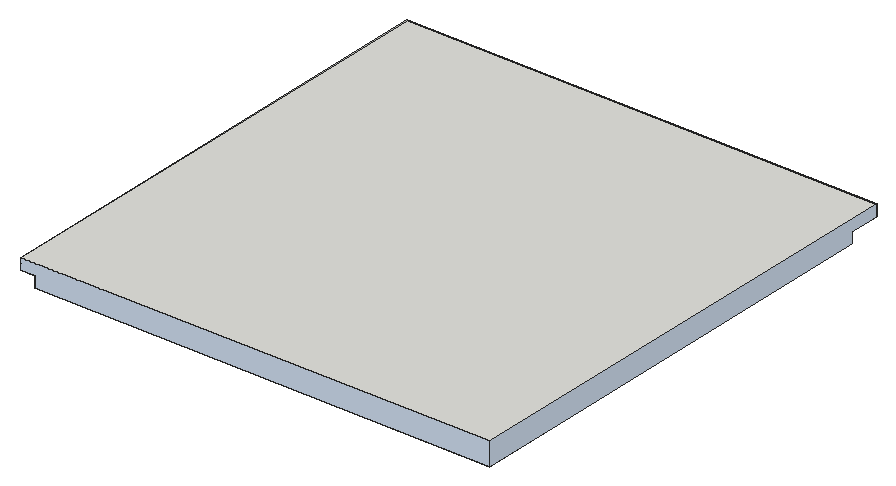
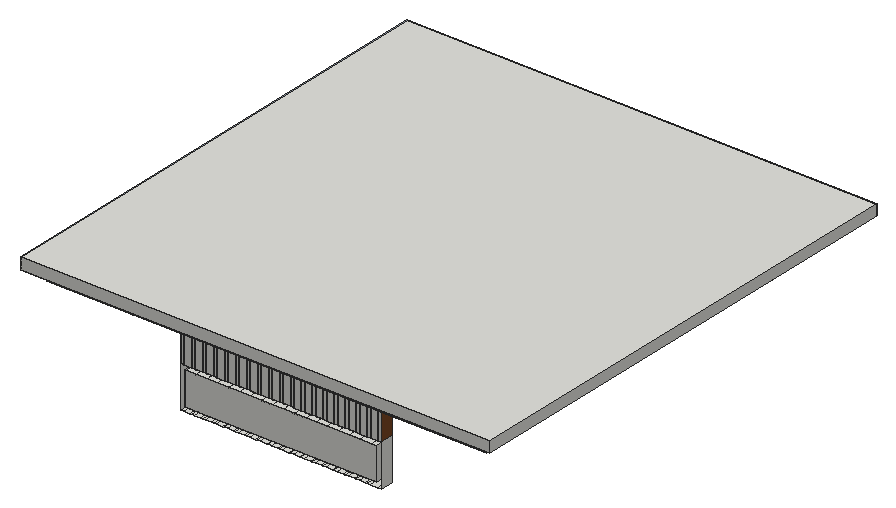
# SketchUp Ruby script. Lengths in inches.
U = 1.inch
M = Sketchup.active_model
def pt(a) = Geom::Point3d.new(a.map { |v| v * U })
def face(e, loops, mat)
  f = e.add_face(loops[0].map { |a| pt(a) })
  loops[1..].each { |l| e.add_face(l.map { |a| pt(a) }).erase! }
  f.material = f.back_material = mat if mat
  f
end
# faces: each face lists its corners as indices into pts; further lists are holes
def faces(e, pts, list, mat = nil) = list.each { |f| face(e, (f[0].is_a?(Array) ? f : [f]).map { |l| l.map { |i| pts[i] } }, mat) }
# xy, xz, yz: faces in a plane at the given z, y or x. An outline is a flat list of corners, or four numbers for a rectangle; further outlines are holes
def ring(l) = l.size == 4 ? [[l[0], l[1]], [l[2], l[1]], [l[2], l[3]], [l[0], l[3]]] : l.each_slice(2).to_a
def flat(e, list, mat, &to3) = list.each { |f| face(e, (f[0].is_a?(Array) ? f : [f]).map { |l| ring(l).map { |u, v| to3.(u, v) } }, mat) }
def xy(e, z, list, mat = nil) = flat(e, list, mat) { |x, y| [x, y, z] }
def xz(e, y, list, mat = nil) = flat(e, list, mat) { |x, z| [x, y, z] }
def yz(e, x, list, mat = nil) = flat(e, list, mat) { |y, z| [x, y, z] }
def lines(e, pts, list) = list.each { |a, b| e.add_line(pt(pts[a]), pt(pts[b])) }
# prism: a flat outline (further loops are holes) pulled along v
def prism(e, loops, v, mat = nil)
  f = face(e, loops, mat); d = Geom::Vector3d.new(v.map { |x| x * U })
  f.pushpull(f.normal.samedirection?(d) ? d.length : -d.length)
end
def box(e, o, s, mat = nil) = prism(e, [[o, [o[0] + s[0], o[1], o[2]], [o[0] + s[0], o[1] + s[1], o[2]], [o[0], o[1] + s[1], o[2]]]], [0, 0, s[2]], mat)
def at(x, y, z, deg = 0) = Geom::Transformation.translation(pt([x, y, z])) * Geom::Transformation.rotation(ORIGIN, Z_AXIS, deg.degrees)
def axes(o, x, y, z) = Geom::Transformation.new([*x, 0, *y, 0, *z, 0, *pt(o).to_a, 1])
def part(name) = M.definitions.add(name)
# library, detail: a bought-in or finely detailed component or shape, given as its bounding box
def library(name, o, s) = part(name).tap { |d| box(d.entities, o, s) }
def detail(e, o, s) = box(e.add_group.entities, o, s)
def put(e, d, t, mat = nil) = e.add_instance(d, t).tap { |i| i.material = mat if mat }
def group(e, t, mat = nil) = e.add_group.tap { |g| g.transformation = t; g.material = mat if mat }.entities
root = M.entities
M.materials.add("Generic").color = [214, 229, 247]
M.materials.add("[Wood Veneer 01]").color = [120, 70, 37]
M.materials.add("hymenocallis littoralis").color = [156, 172, 146]
c1 = part("Group\#856")
xy(c1.entities,7.38,[[0,0,5.5,15.91]],"hymenocallis littoralis")
p = [[5.5,28.78,0],[5.5,26.79,3.44],[0,26.79,3.44],[0,28.78,0],[0,23.75,6],[5.5,23.75,6],
  [0,15.91,7.38],[5.5,15.91,7.38]]
faces(c1.entities,p,[[0,1,2,3],[4,2,1,5],[6,4,5,7]],"hymenocallis littoralis")
c2 = part("Group\#854")
xy(c2.entities,7.38,[[0,0,5.5,15.91],[0,15.91,5.5,23.87]],"hymenocallis littoralis")
p = [[5.5,31.07,4.3],[5.5,27.74,6.47],[0,27.74,6.47],[0,31.07,4.3],[0,23.87,7.38],[5.5,23.87,7.38]]
faces(c2.entities,p,[[0,1,2,3],[4,2,1,5]],"hymenocallis littoralis")
c3 = part("Group\#857")
xy(c3.entities,7.38,[[0,0,5.6,15.91]],"hymenocallis littoralis")
p = [[5.6,28.78,0],[5.6,26.79,3.44],[0,26.79,3.44],[0,28.78,0],[0,23.75,6],[5.6,23.75,6],
  [0,15.91,7.38],[5.6,15.91,7.38]]
faces(c3.entities,p,[[0,1,2,3],[4,2,1,5],[6,4,5,7]],"hymenocallis littoralis")
c4 = part("Group\#855")
put(c4.entities,c2,axes([6.09,8.57,-0.52],[0.446,0.85617,0.26089],[-0.18444,-0.19731,0.96283],[0.87582,-0.47754,0.0699]))
put(c4.entities,c2,axes([6.29,7.28,-1.71],[0.37058,0.92707,-0.05667],[-0.32382,0.19004,0.99128],[0.87712,-0.32925,0.34964]))
put(c4.entities,c2,axes([11.04,16.14,-0.7],[1,0,0],[0,0.16628,1.02662],[0,-1.18456,0.19186]))
c5 = part("Group\#860")
put(c5.entities,c1,axes([24.57,32.05,-1.76],[0.9552,-0.22102,-0.19681],[0.4036,0.95545,0.88585],[-0.00568,-0.67859,0.7345]))
put(c5.entities,c1,axes([23.95,29.24,-2.4],[0,1,0],[-0.76041,0,0.64945],[0.64945,0,0.76041]))
put(c5.entities,c1,axes([24.22,24.72,-0.48],[-0.70711,0.70711,0],[-0.32757,-0.32757,0.80237],[0.61237,0.61237,0.5]))
put(c5.entities,c2,axes([20.66,37.22,-0.63],[1.12361,0.03262,0.39091],[-0.43499,0.29739,0.78777],[0.09852,-1.27434,0.37535]))
put(c5.entities,c1,axes([28.75,24.45,-2.4],[-1,0,0],[0,-0.76041,0.64945],[0,0.64945,0.76041]))
put(c5.entities,c3,axes([30.4,30.98,-3.7],[0.65676,-0.72002,0.22414],[0.55667,0.66341,0.5],[-0.50871,-0.20361,0.83652]))
put(c5.entities,c3,axes([32.41,29.61,-3.7],[0.04029,-0.97372,0.22414],[0.85287,0.15038,0.5],[-0.52057,0.17102,0.83652]))
put(c5.entities,c1,axes([31.89,25.85,-1.76],[-0.92056,0.33739,-0.19681],[-0.5186,-0.89824,0.88585],[0.08952,0.67268,0.7345]))
put(c5.entities,c1,axes([25.55,34.78,-0.48],[0.86603,0.5,0],[-0.25,0.43301,0.86603],[0.43301,-0.75,0.5]))
put(c5.entities,c3,axes([20.4,16.9375,-8.07],[-0.70711,0.70711,0],[-0.35754,-0.35754,0.65422],[1.3987,1.3987,1.52882]))
put(c5.entities,c1,axes([32.86,34.14,-0.48],[0.76604,-0.64279,0],[0.32139,0.38302,0.86603],[-0.55667,-0.66341,0.5]))
put(c5.entities,c1,axes([27.15,34.7,-0.1],[0.82472,-0.17528,-0.53769],[0.53769,0.53769,0.64945],[0.17528,-0.82472,0.53769]))
put(c5.entities,c1,axes([33.58,28.77,-2.4],[0,-1,0],[0.76041,0,0.64945],[-0.64945,0,0.76041]))
put(c5.entities,c1,axes([26.43,23.87,-2.81],[-0.75126,0.04415,0.65853],[0.53769,-0.53769,0.64945],[0.38276,0.84199,0.3802]))
put(c5.entities,c1,axes([28.78,23.98,-2.4],[-1,0,0],[0,-0.76041,0.64945],[0,0.64945,0.76041]))
put(c5.entities,c1,axes([25.39,25.38,-2.4],[-0.70711,0.70711,0],[-0.53769,-0.53769,0.64945],[0.45923,0.45923,0.76041]))
put(c5.entities,c1,axes([27.32,21.63,-0.1],[-0.45923,0.70711,-0.53769],[-0.76041,0,0.64945],[0.45923,0.70711,0.53769]))
put(c5.entities,c1,axes([25.17,27.625,-1.76],[0.56416,0.80187,-0.19681],[-0.66673,0.66673,0.80532],[0.62659,-0.26057,0.7345]))
put(c5.entities,c3,axes([27.59,27.04,-3.96],[-0.8993,-0.06127,0.43301],[0.2962,-0.8138,0.5],[0.32175,0.57791,0.75]))
put(c5.entities,c3,axes([26.98,24.5,-3.18],[-0.5,0.86603,0],[-0.75,-0.43301,0.5],[0.43301,0.25,0.86603]))
put(c5.entities,c3,axes([24.55,27.74,-3.7],[0.29517,0.92878,0.22414],[-0.85287,0.15038,0.5],[0.43068,-0.33875,0.83652]))
put(c5.entities,c3,axes([24.26,29.8,-3.18],[0.76604,0.64279,0],[-0.47317,0.5639,0.425],[0.32139,-0.38302,0.86603]))
put(c5.entities,c3,axes([25.98,32.46,-3.18],[1,0,0],[0,0.86603,0.5],[0,-0.5,0.86603]))
put(c5.entities,c1,axes([28.78,33.57,-2.4],[1,0,0],[0,0.76041,0.64945],[0,-0.64945,0.76041]))
put(c5.entities,c4,at(14.99,21.38,2.5))
put(c5.entities,c2,axes([34.63,26.34,-1.46],[-0.70089,-0.70877,0.07994],[0.4756,-0.38088,0.79293],[-0.53156,0.59378,0.60405]))
put(c5.entities,c2,axes([28.14,16.92,1.8125],[-1.19719,0.6912,0],[-0.09607,-0.16641,0.94244],[0.68444,1.18549,0.17613]))
put(c5.entities,c2,axes([31.5625,35.84,0.97],[0.66765,-1.1564,0.35779],[0.04445,0.30732,0.91033],[-1.20828,-0.64496,0.17012]))
put(c5.entities,c2,axes([38.94,22.51,0.89],[-0.97932,-0.67164,-0.05202],[0.27787,-0.41401,0.90999],[-0.85985,0.93577,0.32097]))
put(c5.entities,c2,axes([38.44,21.09,1.98],[-1.02864,-0.54856,0.2395],[0.33481,0.06999,0.88388],[-0.77261,1.08328,0.06417]))
put(c5.entities,c3,axes([35.02,30.51,-1.3],[-0.17365,-0.98481,0],[0.60224,-0.10619,0.79122],[-0.7792,0.13739,0.61153]))
put(c5.entities,c3,axes([29.41,22.33,-1.3],[-0.93969,0.34202,0],[-0.20915,-0.57465,0.79122],[0.27061,0.74351,0.61153]))
put(c5.entities,c2,axes([19.64,36,-1.62],[1.18194,0.09546,0.08234],[-0.14377,0.68823,0.76313],[0.21457,-1.1326,0.62386]))
put(c5.entities,c3,axes([24.25,24.14,-1.3],[-0.34202,0.93969,0],[-0.57465,-0.20915,0.79122],[0.74351,0.27061,0.61153]))
put(c5.entities,c3,axes([25.98,34.61,-1.3],[1,0,0],[0,0.61153,0.79122],[0,-0.79122,0.61153]))
put(c5.entities,c3,axes([31.16,34.41,-1.64],[0.56518,-0.80224,-0.19234],[0.73413,0.34233,0.72935],[-0.47639,-0.50772,0.71782]))
put(c5.entities,c3,axes([40.52,26.84,-5.82],[-0.42262,-0.90631,0],[0.48019,-0.22391,0.68552],[-1.43418,0.66877,1.22305]))
put(c5.entities,c1,axes([29.86,38.42,-1.01],[0.89064,-0.37013,0.26413],[-0.03924,0.63286,1.01918],[-0.45353,-0.76487,0.45748]))
put(c5.entities,c1,axes([29.34,22.4,-0.48],[-0.99619,-0.08716,0],[0.04358,-0.4981,0.86603],[-0.07548,0.86273,0.5]))
c6 = part("Group\#858")
xz(c6.entities,10.07,[[9.07,0,10.07,31.01],[0,31.01,0,45.12,20.13,45.12,20.13,31.01,10.07,31.01,10.07,32.58,9.07,32.58,9.07,31.01]],"hymenocallis littoralis")
yz(c6.entities,10.07,[[0,31.01,20.13,45.12]],"hymenocallis littoralis")
p = [[9.57,9.2,0],[10.07,10.07,0],[10.07,10.07,31.01],[10.07,10.07,32.58],[9.57,9.2,32.58]]
faces(c6.entities,p,[[0,1,2,3,4]],"hymenocallis littoralis")
c7 = part("cây lá nắng")
put(c7.entities,c5,axes([49.26,-2.75,0],[0.63109,0.63109,0],[-0.63109,0.63109,0],[0,0,0.935]))
g1 = group(c7.entities,at(26.6,-8.68,0))
put(g1,c1,axes([-4.72,35.73,-1.65],[0.74231,0.46334,-0.18402],[-0.34827,0.85768,0.82827],[0.42467,-0.43184,0.68675]))
put(g1,c1,axes([-3.34,33.57,-2.24],[-0.63109,0.63109,0],[-0.47989,-0.47989,0.60723],[0.40986,0.40986,0.71098]))
put(g1,c1,axes([-0.3125,30.89,-0.45],[-0.8925,0,0],[0,-0.41345,0.75022],[0,0.77293,0.4675]))
put(g1,c2,axes([-10.79,39.66,-0.59],[0.68852,0.72969,0.3655],[-0.4622,-0.08684,0.73657],[0.86641,-0.74205,0.35095]))
put(g1,c1,axes([2.71,33.57,-2.24],[-0.63109,-0.63109,0],[0.47989,-0.47989,0.60723],[-0.40986,0.40986,0.71098]))
put(g1,c3,axes([-0.37,38.74,-3.46],[0.86887,-0.03992,0.20957],[-0.06737,0.76999,0.4675],[-0.19255,-0.44954,0.78214]))
put(g1,c3,axes([1.76,39.14,-3.46],[0.63993,-0.58908,0.20957],[0.44333,0.63315,0.4675],[-0.43646,-0.2206,0.78214]))
put(g1,c1,axes([3.81,36.4375,-1.65],[-0.79389,-0.36803,-0.18402],[0.23959,-0.89415,0.82827],[-0.36803,0.48102,0.68675]))
put(g1,c1,axes([-5.83,38.07,-0.45],[0.231,0.86209,0],[-0.43104,0.1155,0.80973],[0.74659,-0.20005,0.4675]))
put(g1,c3,axes([2.18,23.5625,-7.55],[-0.8925,0,0],[0,-0.45128,0.6117],[0,1.76542,1.42944]))
put(g1,c1,axes([-0.8125,42.28,-0.45],[0.8891,0.07779,0],[-0.03889,0.44455,0.80973],[0.06737,-0.76999,0.4675]))
put(g1,c1,axes([-4.76,39.03,-0.09],[0.63109,0.40986,-0.50274],[0,0.67866,0.60723],[0.63109,-0.40986,0.50274]))
put(g1,c1,axes([3.03,39.35,-2.24],[0.63109,-0.63109,0],[0.47989,0.47989,0.60723],[-0.40986,-0.40986,0.71098]))
put(g1,c1,axes([1.61,31.74,-2.625],[-0.50198,-0.44625,0.61573],[0.67866,0,0.60723],[-0.28982,0.77293,0.35549]))
put(g1,c1,axes([3.03,33.3,-2.24],[-0.63109,-0.63109,0],[0.47989,-0.47989,0.60723],[-0.40986,0.40986,0.71098]))
put(g1,c1,axes([0.01,32.04,-2.24],[-0.8925,0,0],[0,-0.67866,0.60723],[0,0.57963,0.71098]))
put(g1,c1,axes([3.59,30.89,-0.09],[-0.73607,0.15643,-0.50274],[-0.47989,-0.47989,0.60723],[-0.15643,0.73607,0.50274]))
put(g1,c1,axes([-1.55,33.32,-1.65],[-0.15002,0.86209,-0.18402],[-0.84154,0,0.75297],[0.55988,0.231,0.68675]))
put(g1,c3,axes([0.35,34.48,-3.71],[-0.52887,-0.60621,0.40487],[0.70051,-0.32665,0.4675],[-0.16166,0.56777,0.70125]))
put(g1,c3,axes([2.61,39.13,-1.74],[-0.86209,0.231,0],[-0.23031,-0.85954,0.15531],[0.03162,0.11799,0.91645]))
put(g1,c3,axes([-2.02,33,-3.46],[-0.39986,0.77243,0.20957],[-0.63315,-0.44333,0.4675],[0.48558,0.05802,0.78214]))
put(g1,c3,axes([-3.49,34.12,-2.97],[0.07779,0.8891,0],[-0.65449,0.05726,0.39737],[0.44455,-0.03889,0.80973]))
put(g1,c3,axes([-4.09,36.88,-2.97],[0.63109,0.63109,0],[-0.54654,0.54654,0.4675],[0.31555,-0.31555,0.80973]))
put(g1,c1,axes([-3.02,39.35,-2.24],[0.63109,0.63109,0],[-0.47989,0.47989,0.60723],[0.40986,-0.40986,0.71098]))
put(g1,c4,axes([-4.03,22.95,2.33],[0.63109,0.63109,0],[-0.63109,0.63109,0],[0,0,0.935]))
put(g1,c2,axes([5.24,38.48,-1.37],[0.00497,-0.88963,0.07474],[0.54052,0.05978,0.74139],[-0.71019,0.03927,0.56479]))
put(g1,c2,axes([7.08,28.4375,1.7],[-1.19175,-0.31933,0],[0.04439,-0.16565,0.88118],[-0.31621,1.1801,0.16468]))
put(g1,c2,axes([-2.7,42.54,0.91],[1.15114,-0.30845,0.33454],[-0.1659,0.22199,0.85115],[-0.3555,-1.16957,0.15907]))
put(g1,c2,axes([10.37,38.78,0.83],[-0.19417,-1.04191,-0.04864],[0.43664,-0.08592,0.85084],[-1.1332,0.04791,0.30011]))
put(g1,c2,axes([10.95,37.5625,1.85],[-0.30298,-0.99536,0.22393],[0.16713,0.25547,0.82643],[-1.17124,0.19607,0.06]))
put(g1,c3,axes([2.84,41.36,-1.22],[0.51192,-0.73109,0],[0.44708,0.31305,0.73979],[-0.57846,-0.40504,0.57178]))
put(g1,c3,axes([4.47,32.65,-1.22],[-0.80888,-0.37719,0],[0.23066,-0.49465,0.73979],[-0.29844,0.64,0.57178]))
put(g1,c2,axes([-10.32,35.12,-1.51],[0.68567,0.80616,0.07699],[-0.52507,0.3436,0.71352],[0.85019,-0.57936,0.58331]))
put(g1,c3,axes([0.07,30.54,-1.22],[-0.80888,0.37719,0],[-0.23066,-0.49465,0.73979],[0.29844,0.64,0.57178]))
put(g1,c3,axes([-5.45,38.24,-1.22],[0.63109,0.63109,0],[-0.38593,0.38593,0.73979],[0.49934,-0.49934,0.57178]))
put(g1,c3,axes([-2.05,41.38,-1.53],[0.86296,-0.14961,-0.17984],[0.24726,0.67935,0.68194],[0.01977,-0.62107,0.67116]))
put(g1,c3,axes([8.63,42.51,-5.4375],[0.30525,-0.83868,0],[0.44435,0.16173,0.64096],[-1.32716,-0.48305,1.14356]))
put(g1,c1,axes([-5.4,43.09,-0.94],[0.79566,0.32849,0.24696],[-0.42416,0.37462,0.95293],[0.19648,-0.76892,0.42774]))
put(g1,c1,axes([4.38,32.65,-0.45],[-0.57369,-0.68369,0],[0.34185,-0.28684,0.80973],[-0.5921,0.49683,0.4675]))
put(g1,c3,axes([-2,33.84,-0.15],[-0.24601,0.85793,0],[-0.85539,-0.24528,0.15531],[0.11742,0.03367,0.91645]))
put(g1,c3,axes([0.17,30.83,-4.47],[-0.24601,0.85793,0],[-0.85539,-0.24528,0.15531],[0.11742,0.03367,0.91645]))
put(g1,c3,axes([-1.97,32.18,-4.47],[0.58524,0.67383,0],[-0.67184,0.58351,0.15531],[0.09222,-0.0801,0.91645]))
put(g1,c3,axes([-2,34.71,-4.47],[0.88392,-0.12346,0],[0.12309,0.88131,0.15531],[-0.0169,-0.12098,0.91645]))
put(g1,c3,axes([0.11,36.12,-4.47],[0.37822,-0.8084,0],[0.80601,0.37711,0.15531],[-0.11064,-0.05177,0.91645]))
put(c7.entities,c6,axes([29.71,14.29,6.94],[0.425,0.73612,0],[-0.6771,0.39092,-0.33349],[-0.26859,0.15507,0.72712]))
put(c7.entities,c6,axes([42.0625,26.12,6.94],[0.85,0,0],[0,0.78185,-0.33349],[0,0.33349,0.78185]))
put(c7.entities,c5,axes([7.3125,23.0625,0],[0.8925,0,0],[0,0.8925,0],[0,0,0.935]))
put(c7.entities,c6,axes([24.4375,40.23,2.05],[0.85,0,0],[0,0.85,0],[0,0,0.85]))
c8 = part("Planting+101")
put(c8.entities,c7,axes([21.34,32.96,-4.59],[0,-0.71,0],[-0.71,0,0],[0,0,0.71]))
xy(root,125.75,[[108.4375,360.5625,111,370.9375],[111,360.5625,117.4375,370.9375],[117.4375,360.5625,120,370.9375],[120,360.5625,121.24,370.9375],[121.24,360.5625,126.4375,370.9375],
  [126.4375,360.5625,129,370.9375],[129,360.5625,130.24,370.9375],[130.24,360.5625,135.4375,370.9375],[135.4375,360.5625,138,370.9375],[138,360.5625,139.24,370.9375],
  [139.24,360.5625,144.4375,370.9375],[144.4375,360.5625,147,370.9375],[147,360.5625,148.24,370.9375],[148.24,360.5625,153.4375,370.9375],[153.4375,360.5625,156,370.9375],
  [156,360.5625,157.24,370.9375],[157.24,360.5625,162.4375,370.9375],[162.4375,360.5625,165,370.9375],[165,360.5625,166.24,370.9375],[166.24,360.5625,171.4375,370.9375],
  [171.4375,360.5625,174,370.9375],[174,360.5625,175.24,370.9375],[175.24,360.5625,180.4375,370.9375],[180.4375,360.5625,183,370.9375],[183,360.5625,184.24,370.9375],
  [184.24,360.5625,189.4375,370.9375],[189.4375,360.5625,192,370.9375],[192,360.5625,193.24,370.9375],[193.24,360.5625,198.4375,370.9375],[198.4375,360.5625,201,370.9375],
  [201,360.5625,202.24,370.9375],[202.24,360.5625,207.4375,370.9375],[207.4375,360.5625,210,370.9375],[210,360.5625,211.24,370.9375],[211.24,360.5625,216.4375,370.9375],
  [216.4375,360.5625,219,370.9375],[219,360.5625,220.24,370.9375],[220.24,360.5625,225.4375,370.9375],[225.4375,360.5625,228,370.9375],[228,360.5625,229.24,370.9375],
  [229.24,360.5625,234.4375,370.9375],[234.4375,360.5625,237,370.9375],[237,360.5625,238.24,370.9375],[238.24,360.5625,243.4375,370.9375],[243.4375,360.5625,246,370.9375],
  [246,360.5625,247.24,370.9375],[247.24,360.5625,252.4375,370.9375],[252.4375,360.5625,255,370.9375],[255,360.5625,256.24,370.9375],[256.24,360.5625,261.4375,370.9375],
  [261.4375,360.5625,264,370.9375],[264,360.5625,265.24,370.9375],[265.24,360.5625,270.4375,370.9375],[270.4375,360.5625,273,370.9375]])
xy(root,129.55,[[112.24,360.5625,121.24,370.9375],[121.24,360.5625,130.24,370.9375],[130.24,360.5625,139.24,370.9375],[139.24,360.5625,148.24,370.9375],[148.24,360.5625,157.24,370.9375],
  [157.24,360.5625,166.24,370.9375],[166.24,360.5625,175.24,370.9375],[175.24,360.5625,184.24,370.9375],[184.24,360.5625,193.24,370.9375],[193.24,360.5625,202.24,370.9375],
  [202.24,360.5625,211.24,370.9375],[211.24,360.5625,220.24,370.9375],[220.24,360.5625,229.24,370.9375],[229.24,360.5625,238.24,370.9375],[238.24,360.5625,247.24,370.9375],
  [247.24,360.5625,256.24,370.9375],[256.24,360.5625,265.24,370.9375],[265.24,360.5625,269.2,370.9375]])
xy(root,156.13,[[112.24,360.5625,116.2,370.9375],[116.2,360.5625,125.2,370.9375],[125.2,360.5625,134.2,370.9375],[134.2,360.5625,143.2,370.9375],[143.2,360.5625,152.2,370.9375],
  [152.2,360.5625,161.2,370.9375],[161.2,360.5625,170.2,370.9375],[170.2,360.5625,179.2,370.9375],[179.2,360.5625,188.2,370.9375],[188.2,360.5625,197.2,370.9375],
  [197.2,360.5625,206.2,370.9375],[206.2,360.5625,215.2,370.9375],[215.2,360.5625,224.2,370.9375],[224.2,360.5625,233.2,370.9375],[233.2,360.5625,242.2,370.9375],
  [242.2,360.5625,251.2,370.9375],[251.2,360.5625,260.2,370.9375],[260.2,360.5625,269.2,370.9375]])
xy(root,159.9375,[[108.4375,360.5625,111,370.9375],[111,360.5625,116.2,370.9375],[116.2,360.5625,117.4375,370.9375],[117.4375,360.5625,120,370.9375],[120,360.5625,125.2,370.9375],
  [125.2,360.5625,126.4375,370.9375],[126.4375,360.5625,129,370.9375],[129,360.5625,134.2,370.9375],[134.2,360.5625,135.4375,370.9375],[135.4375,360.5625,138,370.9375],
  [138,360.5625,143.2,370.9375],[143.2,360.5625,144.4375,370.9375],[144.4375,360.5625,147,370.9375],[147,360.5625,152.2,370.9375],[152.2,360.5625,153.4375,370.9375],
  [153.4375,360.5625,156,370.9375],[156,360.5625,161.2,370.9375],[161.2,360.5625,162.4375,370.9375],[162.4375,360.5625,165,370.9375],[165,360.5625,170.2,370.9375],
  [170.2,360.5625,171.4375,370.9375],[171.4375,360.5625,174,370.9375],[174,360.5625,179.2,370.9375],[179.2,360.5625,180.4375,370.9375],[180.4375,360.5625,183,370.9375],
  [183,360.5625,188.2,370.9375],[188.2,360.5625,189.4375,370.9375],[189.4375,360.5625,192,370.9375],[192,360.5625,197.2,370.9375],[197.2,360.5625,198.4375,370.9375],
  [198.4375,360.5625,201,370.9375],[201,360.5625,206.2,370.9375],[206.2,360.5625,207.4375,370.9375],[207.4375,360.5625,210,370.9375],[210,360.5625,215.2,370.9375],
  [215.2,360.5625,216.4375,370.9375],[216.4375,360.5625,219,370.9375],[219,360.5625,224.2,370.9375],[224.2,360.5625,225.4375,370.9375],[225.4375,360.5625,228,370.9375],
  [228,360.5625,233.2,370.9375],[233.2,360.5625,234.4375,370.9375],[234.4375,360.5625,237,370.9375],[237,360.5625,242.2,370.9375],[242.2,360.5625,243.4375,370.9375],
  [243.4375,360.5625,246,370.9375],[246,360.5625,251.2,370.9375],[251.2,360.5625,252.4375,370.9375],[252.4375,360.5625,255,370.9375],[255,360.5625,260.2,370.9375],
  [260.2,360.5625,261.4375,370.9375],[261.4375,360.5625,264,370.9375],[264,360.5625,270.4375,370.9375],[270.4375,360.5625,273,370.9375]])
xy(root,191.375,[[[12,0,12,384,372,384,372,370.9375,384,370.9375,384,0],[110.625,35.16,144.4375,319.91],[162.6875,35.16,196.5,319.91],[214.75,35.16,248.5625,319.91],[266.8125,35.16,300.625,319.91],[58.5625,35.16,92.375,319.91]]],"Generic")
xy(root,192,[[12,113.46,27,168.59],[12,314.25,27,370.9375],[27,314.25,40.0625,317.625],[84,360.5625,90.4375,370.9375],[93,360.5625,99.4375,370.9375],
  [102,360.5625,108.4375,370.9375],[111,360.5625,117.4375,370.9375],[120,360.5625,126.4375,370.9375],[129,360.5625,135.4375,370.9375],[138,360.5625,144.4375,370.9375],
  [147,360.5625,153.4375,370.9375],[156,360.5625,162.4375,370.9375],[165,360.5625,171.4375,370.9375],[174,360.5625,180.4375,370.9375],[183,360.5625,189.4375,370.9375],
  [192,360.5625,198.4375,370.9375],[201,360.5625,207.4375,370.9375],[210,360.5625,216.4375,370.9375],[219,360.5625,225.4375,370.9375],[228,360.5625,234.4375,370.9375],
  [237,360.5625,243.4375,370.9375],[246,360.5625,252.4375,370.9375],[255,360.5625,261.4375,370.9375],[264,360.5625,270.4375,370.9375],[273,360.5625,279.4375,370.9375],
  [282,360.5625,288.4375,370.9375],[291,360.5625,297.4375,370.9375],[12,370.9375,84,384],[84,370.9375,300,384],[300,370.9375,372,384]])
xy(root,200.8125,[[0,0,12,113.46],[0,113.46,12,170.15],[0,170.15,12,314.25],[0,314.25,12,370.9375],[0,370.9375,0,396,84,396,84,384,12,384,12,370.9375],
  [372,370.9375,372,384,300,384,300,396,384,396,384,370.9375],[84,384,300,396]])
xy(root,202.4375,[[58.5625,35.16,92.375,319.91],[110.625,35.16,144.4375,319.91],[162.6875,35.16,196.5,319.91],[214.75,35.16,248.5625,319.91],[266.8125,35.16,300.625,319.91]])
xy(root,209.8125,[[0,0,384,396]])
xz(root,0,[[12,191.375,384,191.375,384,209.8125,0,209.8125,0,200.8125,12,200.8125]],"Generic")
xz(root,35.16,[[58.5625,191.375,92.375,202.4375],[110.625,191.375,144.4375,202.4375],[162.6875,191.375,196.5,202.4375],[214.75,191.375,248.5625,202.4375],[266.8125,191.375,300.625,202.4375]])
xz(root,319.91,[[58.5625,191.375,92.375,202.4375],[110.625,191.375,144.4375,202.4375],[162.6875,191.375,196.5,202.4375],[214.75,191.375,248.5625,202.4375],[266.8125,191.375,300.625,202.4375]])
xz(root,360.5625,[[[108.4375,125.75,273,159.9375],[112.24,129.55,269.2,156.13]],[111,159.9375,117.4375,192],[120,159.9375,126.4375,192],[129,159.9375,135.4375,192],[138,159.9375,144.4375,192],
  [147,159.9375,153.4375,192],[156,159.9375,162.4375,192],[165,159.9375,171.4375,192],[174,159.9375,180.4375,192],[183,159.9375,189.4375,192],
  [192,159.9375,198.4375,192],[201,159.9375,207.4375,192],[210,159.9375,216.4375,192],[219,159.9375,225.4375,192],[228,159.9375,234.4375,192],
  [237,159.9375,243.4375,192],[246,159.9375,252.4375,192],[255,159.9375,261.4375,192],[264,159.9375,270.4375,192]],"[Wood Veneer 01]")
xz(root,370.9375,[[112.24,129.55,269.2,156.13],[108.4375,159.9375,111,192],[111,159.9375,117.4375,192],[117.4375,159.9375,120,192],[120,159.9375,126.4375,192],
  [126.4375,159.9375,129,192],[129,159.9375,135.4375,192],[135.4375,159.9375,138,192],[138,159.9375,144.4375,192],[144.4375,159.9375,147,192],
  [147,159.9375,153.4375,192],[153.4375,159.9375,156,192],[156,159.9375,162.4375,192],[162.4375,159.9375,165,192],[165,159.9375,171.4375,192],
  [171.4375,159.9375,174,192],[174,159.9375,180.4375,192],[180.4375,159.9375,183,192],[183,159.9375,189.4375,192],[189.4375,159.9375,192,192],
  [192,159.9375,198.4375,192],[198.4375,159.9375,201,192],[201,159.9375,207.4375,192],[207.4375,159.9375,210,192],[210,159.9375,216.4375,192],
  [216.4375,159.9375,219,192],[219,159.9375,225.4375,192],[225.4375,159.9375,228,192],[228,159.9375,234.4375,192],[234.4375,159.9375,237,192],
  [237,159.9375,243.4375,192],[243.4375,159.9375,246,192],[246,159.9375,252.4375,192],[252.4375,159.9375,255,192],[255,159.9375,261.4375,192],
  [261.4375,159.9375,264,192],[264,159.9375,270.4375,192],[270.4375,159.9375,273,192],[372,191.375,384,200.8125]])
xz(root,384,[[12,191.375,84,192],[84,191.375,300,192],[300,191.375,372,192],[12,192,84,200.8125],[84,192,300,200.8125],
  [300,192,372,200.8125]])
xz(root,396,[[0,200.8125,384,209.8125]])
yz(root,0,[[0,200.8125,396,209.8125]])
yz(root,12,[[0,191.375,113.46,200.8125],[113.46,191.375,168.59,192],[168.59,191.375,170.15,200.8125],[170.15,191.375,314.25,200.8125],[314.25,191.375,370.9375,192],
  [370.9375,191.375,384,192],[113.46,192,168.59,200.8125],[314.25,192,370.9375,200.8125],[370.9375,192,384,200.8125]])
yz(root,58.5625,[[35.16,191.375,319.91,202.4375]])
yz(root,92.375,[[35.16,191.375,319.91,202.4375]])
yz(root,108.4375,[[360.5625,125.75,370.9375,159.9375]])
yz(root,108.4375,[[360.5625,159.9375,370.9375,192]],"[Wood Veneer 01]")
yz(root,110.625,[[35.16,191.375,319.91,202.4375]])
yz(root,111,[[360.5625,159.9375,370.9375,192]],"[Wood Veneer 01]")
yz(root,112.24,[[360.5625,129.55,370.9375,156.13]])
yz(root,117.4375,[[360.5625,159.9375,370.9375,192]],"[Wood Veneer 01]")
yz(root,120,[[360.5625,159.9375,370.9375,192]],"[Wood Veneer 01]")
yz(root,126.4375,[[360.5625,159.9375,370.9375,192]],"[Wood Veneer 01]")
yz(root,129,[[360.5625,159.9375,370.9375,192]],"[Wood Veneer 01]")
yz(root,135.4375,[[360.5625,159.9375,370.9375,192]],"[Wood Veneer 01]")
yz(root,138,[[360.5625,159.9375,370.9375,192]],"[Wood Veneer 01]")
yz(root,144.4375,[[35.16,191.375,319.91,202.4375]])
yz(root,144.4375,[[360.5625,159.9375,370.9375,192]],"[Wood Veneer 01]")
yz(root,147,[[360.5625,159.9375,370.9375,192]],"[Wood Veneer 01]")
yz(root,153.4375,[[360.5625,159.9375,370.9375,192]],"[Wood Veneer 01]")
yz(root,156,[[360.5625,159.9375,370.9375,192]],"[Wood Veneer 01]")
yz(root,162.4375,[[360.5625,159.9375,370.9375,192]],"[Wood Veneer 01]")
yz(root,162.6875,[[35.16,191.375,319.91,202.4375]])
yz(root,165,[[360.5625,159.9375,370.9375,192]],"[Wood Veneer 01]")
yz(root,171.4375,[[360.5625,159.9375,370.9375,192]],"[Wood Veneer 01]")
yz(root,174,[[360.5625,159.9375,370.9375,192]],"[Wood Veneer 01]")
yz(root,180.4375,[[360.5625,159.9375,370.9375,192]],"[Wood Veneer 01]")
yz(root,183,[[360.5625,159.9375,370.9375,192]],"[Wood Veneer 01]")
yz(root,189.4375,[[360.5625,159.9375,370.9375,192]],"[Wood Veneer 01]")
yz(root,192,[[360.5625,159.9375,370.9375,192]],"[Wood Veneer 01]")
yz(root,196.5,[[35.16,191.375,319.91,202.4375]])
yz(root,198.4375,[[360.5625,159.9375,370.9375,192]],"[Wood Veneer 01]")
yz(root,201,[[360.5625,159.9375,370.9375,192]],"[Wood Veneer 01]")
yz(root,207.4375,[[360.5625,159.9375,370.9375,192]],"[Wood Veneer 01]")
yz(root,210,[[360.5625,159.9375,370.9375,192]],"[Wood Veneer 01]")
yz(root,214.75,[[35.16,191.375,319.91,202.4375]])
yz(root,216.4375,[[360.5625,159.9375,370.9375,192]],"[Wood Veneer 01]")
yz(root,219,[[360.5625,159.9375,370.9375,192]],"[Wood Veneer 01]")
yz(root,225.4375,[[360.5625,159.9375,370.9375,192]],"[Wood Veneer 01]")
yz(root,228,[[360.5625,159.9375,370.9375,192]],"[Wood Veneer 01]")
yz(root,234.4375,[[360.5625,159.9375,370.9375,192]],"[Wood Veneer 01]")
yz(root,237,[[360.5625,159.9375,370.9375,192]],"[Wood Veneer 01]")
yz(root,243.4375,[[360.5625,159.9375,370.9375,192]],"[Wood Veneer 01]")
yz(root,246,[[360.5625,159.9375,370.9375,192]],"[Wood Veneer 01]")
yz(root,248.5625,[[35.16,191.375,319.91,202.4375]])
yz(root,252.4375,[[360.5625,159.9375,370.9375,192]],"[Wood Veneer 01]")
yz(root,255,[[360.5625,159.9375,370.9375,192]],"[Wood Veneer 01]")
yz(root,261.4375,[[360.5625,159.9375,370.9375,192]],"[Wood Veneer 01]")
yz(root,264,[[360.5625,159.9375,370.9375,192]],"[Wood Veneer 01]")
yz(root,266.8125,[[35.16,191.375,319.91,202.4375]])
yz(root,269.2,[[360.5625,129.55,370.9375,156.13]])
yz(root,270.4375,[[360.5625,159.9375,370.9375,192]],"[Wood Veneer 01]")
yz(root,273,[[360.5625,125.75,370.9375,159.9375]])
yz(root,273,[[360.5625,159.9375,370.9375,192]],"[Wood Veneer 01]")
yz(root,300.625,[[35.16,191.375,319.91,202.4375]])
yz(root,372,[[370.9375,191.375,384,192],[370.9375,192,384,200.8125]])
yz(root,384,[[0,191.375,370.9375,191.375,370.9375,200.8125,396,200.8125,396,209.8125,0,209.8125]],"Generic")
put(root,c8,axes([266.75,360.28,148.03],[0,0,0.67981],[-0.833,0,0],[0,-0.48113,0]))
